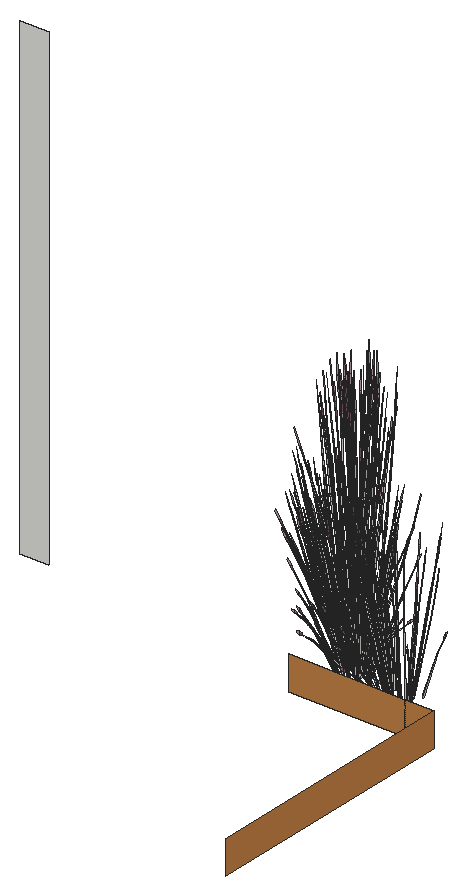
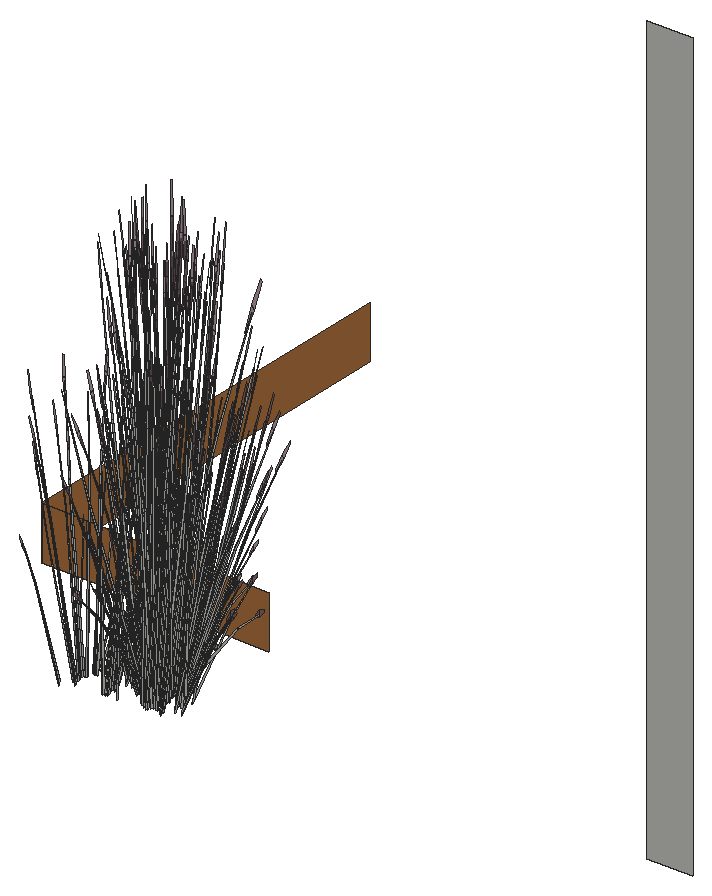
# SketchUp Ruby script. Lengths in inches.
U = 1.inch
M = Sketchup.active_model
def pt(a) = Geom::Point3d.new(a.map { |v| v * U })
def face(e, loops, mat)
  f = e.add_face(loops[0].map { |a| pt(a) })
  loops[1..].each { |l| e.add_face(l.map { |a| pt(a) }).erase! }
  f.material = f.back_material = mat if mat
  f
end
# faces: each face lists its corners as indices into pts; further lists are holes
def faces(e, pts, list, mat = nil) = list.each { |f| face(e, (f[0].is_a?(Array) ? f : [f]).map { |l| l.map { |i| pts[i] } }, mat) }
# xy, xz, yz: faces in a plane at the given z, y or x. An outline is a flat list of corners, or four numbers for a rectangle; further outlines are holes
def ring(l) = l.size == 4 ? [[l[0], l[1]], [l[2], l[1]], [l[2], l[3]], [l[0], l[3]]] : l.each_slice(2).to_a
def flat(e, list, mat, &to3) = list.each { |f| face(e, (f[0].is_a?(Array) ? f : [f]).map { |l| ring(l).map { |u, v| to3.(u, v) } }, mat) }
def xy(e, z, list, mat = nil) = flat(e, list, mat) { |x, y| [x, y, z] }
def xz(e, y, list, mat = nil) = flat(e, list, mat) { |x, z| [x, y, z] }
def yz(e, x, list, mat = nil) = flat(e, list, mat) { |y, z| [x, y, z] }
def lines(e, pts, list) = list.each { |a, b| e.add_line(pt(pts[a]), pt(pts[b])) }
# prism: a flat outline (further loops are holes) pulled along v
def prism(e, loops, v, mat = nil)
  f = face(e, loops, mat); d = Geom::Vector3d.new(v.map { |x| x * U })
  f.pushpull(f.normal.samedirection?(d) ? d.length : -d.length)
end
def box(e, o, s, mat = nil) = prism(e, [[o, [o[0] + s[0], o[1], o[2]], [o[0] + s[0], o[1] + s[1], o[2]], [o[0], o[1] + s[1], o[2]]]], [0, 0, s[2]], mat)
def at(x, y, z, deg = 0) = Geom::Transformation.translation(pt([x, y, z])) * Geom::Transformation.rotation(ORIGIN, Z_AXIS, deg.degrees)
def axes(o, x, y, z) = Geom::Transformation.new([*x, 0, *y, 0, *z, 0, *pt(o).to_a, 1])
def part(name) = M.definitions.add(name)
# library, detail: a bought-in or finely detailed component or shape, given as its bounding box
def library(name, o, s) = part(name).tap { |d| box(d.entities, o, s) }
def detail(e, o, s) = box(e.add_group.entities, o, s)
def put(e, d, t, mat = nil) = e.add_instance(d, t).tap { |i| i.material = mat if mat }
def group(e, t, mat = nil) = e.add_group.tap { |g| g.transformation = t; g.material = mat if mat }.entities
root = M.entities
M.materials.add("LightPink_Translucent").color = [144, 107, 117]
M.materials["LightPink_Translucent"].alpha = 0.75
M.materials.add("Wood_Floor_01_1K").color = [196, 130, 70]
c1 = part("blade")
p = [[2.15,0.21,22],[0,0.17,0],[0.09,0.45,0],[2.18,0.31,22],[2.29,0.31,22],[0.38,0.45,0],
  [2.48,0.24,33],[2.49,0.24,33],[2.48,0.22,33]]
faces(c1.entities,p,[[0,1,2,3],[4,5,2,3],[6,3,4,7],[8,0,3,6]])
c2 = part("seeds")
p = [[0.3,-0.1,1.38],[-0.01,-0.03,1.59],[-0.01,-0.03,0.03],[0.14,-0.07,-0.07],[0.29,-0.03,3],[0.15,0.01,3.11]]
faces(c2.entities,p,[[0,1,2,3],[1,0,4,5]],"LightPink_Translucent")
c3 = part("blade with seeds")
put(c3.entities,c1,at(0,0,0))
put(c3.entities,c2,axes([2.4,0.25,30.99],[1.5799,-0.05474,1.17369],[-0.12525,1.92788,0.29478],[-0.07173,-0.02425,1.56792]))
xz(root,99,[[360,157,384,164],[384,157,390,164]],"Wood_Floor_01_1K")
xz(root,108,[[297,156.54,303,255.54]])
yz(root,390,[[45,157,99,164]],"Wood_Floor_01_1K")
put(root,c3,axes([362.05,110.03,157.34],[0.11194,0.19382,1.61094],[-0.51725,0.16318,0.13026],[-0.1169,-0.30428,0.68866]))
put(root,c3,axes([371.95,108.74,154.43],[-0.0749,-0.08464,1.64448],[-0.49984,0.05366,-0.26007],[-0.07977,-0.20245,0.13189]))
put(root,c3,axes([362.91,108.74,158.13],[-0.0749,-0.08464,1.64448],[-0.49984,0.05366,-0.26007],[-0.07977,-0.20245,0.13189]))
put(root,c3,axes([364.07,109.75,156.13],[-0.13919,0.12219,1.34422],[-0.41687,-0.21387,-0.28909],[0.07727,-0.26598,0.57472]))
put(root,c3,axes([363.43,110.17,158.38],[-0.23372,-0.49086,-0.66783],[0.48111,-0.27356,0.08059],[-0.05465,-0.23717,0.9447]))
put(root,c3,axes([361.91,109.51,156.13],[-0.02965,0.19748,1.34422],[-0.43351,0.16532,-0.28909],[-0.10133,-0.25525,0.57472]))
put(root,c3,axes([363.03,109.08,155.1],[-0.08214,0.02175,1.65762],[-0.45422,-0.24483,-0.25323],[0.00762,-0.20421,0.28235]))
put(root,c3,axes([364.41,110.65,158.38],[0.01274,-0.55841,-0.66783],[0.53656,0.0375,0.08059],[0.05662,-0.23657,0.9447]))
put(root,c3,axes([374.19,109.78,154.43],[-0.00473,-0.12015,1.64448],[-0.39924,-0.34724,-0.26007],[0.06173,-0.21049,0.13189]))
put(root,c3,axes([365.15,109.78,158.13],[-0.00473,-0.12015,1.64448],[-0.39924,-0.34724,-0.26007],[0.06173,-0.21049,0.13189]))
put(root,c3,axes([363.48,109.75,157.95],[0.14763,-0.46424,-0.33289],[0.4307,0.1354,0.42977],[-0.03949,-0.18691,0.82232]))
put(root,c3,axes([363.8,110.37,157.34],[-0.09118,0.2075,1.61094],[-0.3825,-0.42941,0.13026],[0.17255,-0.26763,0.68866]))
put(root,c3,axes([374.09,109.35,154.43],[-0.04973,0.04611,1.6674],[-0.48725,-0.15557,-0.15755],[-0.01764,-0.20123,0.29507]))
put(root,c3,axes([365.05,109.35,158.12],[-0.04973,0.04611,1.6674],[-0.48725,-0.15557,-0.15755],[-0.01764,-0.20123,0.29507]))
put(root,c3,axes([363.26,110.07,158.1],[-0.48137,-0.15133,-0.48033],[0.165,-0.51886,-0.37205],[-0.04414,-0.2089,0.91906]))
put(root,c3,axes([363.56,108.77,156.3],[0.06282,0.35202,1.07969],[-0.34848,-0.19497,0.79328],[0.0375,-0.18025,0.23781]))
put(root,c3,axes([364.3,110.46,158.1],[-0.35055,-0.40562,-0.48033],[0.37031,-0.35523,-0.37205],[0.05334,-0.20609,0.91906]))
put(root,c3,axes([371.4375,108.46,154.43],[-0.00914,0.07236,1.6674],[-0.45057,0.26261,-0.15755],[-0.13259,-0.13424,0.29507]))
put(root,c3,axes([362.4,108.46,158.12],[-0.00914,0.07236,1.6674],[-0.45057,0.26261,-0.15755],[-0.13259,-0.13424,0.29507]))
put(root,c3,axes([371.34,109.75,154.79],[0.5455,-0.15516,0.50537],[0.09467,0.60867,0.4167],[-0.12829,-0.17939,1.04574]))
put(root,c3,axes([362.3,109.75,158.48],[0.5455,-0.15516,0.50537],[0.09467,0.60867,0.4167],[-0.12829,-0.17939,1.04574]))
put(root,c3,axes([372.57,109.86,154.45],[0.48252,0.15782,0.45122],[-0.165,0.51886,0.37205],[-0.029,-0.20404,0.9337]))
put(root,c3,axes([363.53,109.86,158.15],[0.48252,0.15782,0.45122],[-0.165,0.51886,0.37205],[-0.029,-0.20404,0.9337]))
put(root,c3,axes([363.67,110.05,158.43],[-0.47919,0.28106,-0.11431],[-0.23549,-0.49884,-0.63445],[-0.06322,-0.21021,0.96403]))
put(root,c3,axes([364.66,110.68,158.43],[-0.53819,-0.02991,-0.11431],[0.01471,-0.56632,-0.63445],[0.03738,-0.21811,0.96403]))
put(root,c3,axes([364.63,110.31,157.95],[0.33133,-0.31784,-0.33289],[0.31365,0.36292,0.42977],[0.04772,-0.1844,0.82232]))
put(root,c3,axes([361.76,109.2,156.3],[0.25544,0.21011,1.07969],[-0.37201,0.1263,0.79328],[-0.0796,-0.16148,0.23781]))
put(root,c3,axes([372.7,109.82,154.45],[0.36083,-0.20517,0.06044],[0.17661,0.37413,0.47584],[-0.03485,-0.16492,0.72558]))
put(root,c3,axes([363.66,109.82,158.14],[0.36083,-0.20517,0.06044],[0.17661,0.37413,0.47584],[-0.03485,-0.16492,0.72558]))
put(root,c3,axes([362.38,110.31,158.38],[-0.41756,-0.29179,-0.66783],[0.29675,-0.51132,0.08059],[-0.15128,-0.17422,0.9447]))
put(root,c3,axes([362.24,109.92,157.95],[-0.07563,-0.48625,-0.33289],[0.43235,-0.1284,0.42977],[-0.11613,-0.13934,0.82232]))
put(root,c3,axes([371.46,109.88,154.45],[0.22256,-0.38349,0.06044],[0.31694,0.22327,0.47584],[-0.10247,-0.12295,0.72558]))
put(root,c3,axes([362.42,109.88,158.14],[0.22256,-0.38349,0.06044],[0.31694,0.22327,0.47584],[-0.10247,-0.12295,0.72558]))
put(root,c3,axes([361.5625,109.83,155.1],[-0.04743,0.07953,1.65762],[-0.47936,0.17146,-0.25323],[-0.1158,-0.15598,0.28235]))
put(root,c3,axes([361.31,110.63,157.34],[0.1819,0.10401,1.61094],[-0.37643,0.43634,0.13026],[-0.23461,-0.19684,0.68866]))
put(root,c3,axes([365.04,110.12,155.1],[-0.07329,-0.04756,1.65762],[-0.18827,-0.53132,-0.25323],[0.127,-0.14418,0.28235]))
put(root,c3,axes([372.56,110.24,154.75],[-0.14763,0.46424,0.33289],[-0.4307,-0.1354,-0.42977],[-0.03949,-0.18691,0.82232]))
put(root,c3,axes([363.52,110.24,158.44],[-0.14763,0.46424,0.33289],[-0.4307,-0.1354,-0.42977],[-0.03949,-0.18691,0.82232]))
put(root,c3,axes([362.18,110.32,158.1],[-0.48321,0.1435,-0.48033],[-0.08453,-0.54345,-0.37205],[-0.12979,-0.15574,0.91906]))
put(root,c3,axes([373.67,110.4375,154.45],[0.3487,0.41189,0.45122],[-0.37031,0.35523,0.37205],[0.06432,-0.19325,0.9337]))
put(root,c3,axes([364.625,110.4375,158.15],[0.3487,0.41189,0.45122],[-0.37031,0.35523,0.37205],[0.06432,-0.19325,0.9337]))
put(root,c3,axes([371.5625,109.84,155.1],[-0.32682,0.57873,-0.12802],[-0.47329,-0.33342,-0.71058],[-0.16452,-0.16351,1.07972]))
put(root,c3,axes([362.52,109.84,158.8],[-0.32682,0.57873,-0.12802],[-0.47329,-0.33342,-0.71058],[-0.16452,-0.16351,1.07972]))
put(root,c3,axes([373.79,110.48,154.45],[0.40242,0.02813,0.06044],[-0.01103,0.42474,0.47584],[0.04211,-0.1627,0.72558]))
put(root,c3,axes([364.75,110.48,158.14],[0.40242,0.02813,0.06044],[-0.01103,0.42474,0.47584],[0.04211,-0.1627,0.72558]))
put(root,c3,axes([373.49,110.77,154.75],[-0.33133,0.31784,0.33289],[-0.31365,-0.36292,-0.42977],[0.04772,-0.1844,0.82232]))
put(root,c3,axes([364.45,110.77,158.44],[-0.33133,0.31784,0.33289],[-0.31365,-0.36292,-0.42977],[0.04772,-0.1844,0.82232]))
put(root,c3,axes([365.04,111.62,158.38],[0.25579,-0.47633,-0.66783],[0.44823,0.33852,0.08059],[0.15273,-0.17258,0.9447]))
put(root,c3,axes([362.27,110.23,155.93],[-0.30616,-0.60492,0],[0.51222,-0.33735,-0.48511],[0.11666,-0.07683,1.53889]))
put(root,c3,axes([365.03,111.4,158.1],[-0.1258,-0.55122,-0.48033],[0.4764,-0.09643,-0.37205],[0.13652,-0.14806,0.91906]))
put(root,c3,axes([362.95,109.51,155.7],[-0.3384,0.34633,-0.03659],[-0.31006,-0.3793,-0.1659],[-0.02183,-0.10747,0.54722]))
put(root,c3,axes([370.31,109.67,154.43],[-0.10536,-0.00426,1.64448],[-0.33544,0.42612,-0.26007],[-0.17898,-0.08707,0.13189]))
put(root,c3,axes([361.27,109.67,158.13],[-0.10536,-0.00426,1.64448],[-0.33544,0.42612,-0.26007],[-0.17898,-0.08707,0.13189]))
put(root,c3,axes([365.25,111.79,158.43],[-0.45297,-0.33287,-0.11431],[0.26096,-0.48206,-0.63445],[0.12798,-0.16757,0.96403]))
put(root,c3,axes([363.38,113.61,156.82],[0.42317,0.24343,1.42185],[-0.41456,0.52443,0.56227],[-0.18569,-0.31082,1.19198]))
put(root,c3,axes([371.53,110.32,154.75],[0.07563,0.48625,0.33289],[-0.43235,0.1284,-0.42977],[-0.11613,-0.13934,0.82232]))
put(root,c3,axes([362.49,110.32,158.44],[0.07563,0.48625,0.33289],[-0.43235,0.1284,-0.42977],[-0.11613,-0.13934,0.82232]))
put(root,c3,axes([365.41,111.18,156.13],[-0.17494,-0.01788,1.34422],[-0.17922,-0.47967,-0.28909],[0.21491,-0.13569,0.57472]))
put(root,c3,axes([370.23,110.64,154.79],[0.4044,-0.44551,0.50537],[0.34877,0.47312,0.4167],[-0.18973,-0.08218,1.04574]))
put(root,c3,axes([361.19,110.64,158.48],[0.4044,-0.44551,0.50537],[0.34877,0.47312,0.4167],[-0.18973,-0.08218,1.04574]))
put(root,c3,axes([375.41,111.65,154.43],[-0.06396,-0.00458,1.6674],[-0.2656,-0.49127,-0.15755],[0.10666,-0.16153,0.29507]))
put(root,c3,axes([366.37,111.65,158.12],[-0.06396,-0.00458,1.6674],[-0.2656,-0.49127,-0.15755],[0.10666,-0.16153,0.29507]))
put(root,c3,axes([365.61,110.3,156.3],[-0.16311,0.3073,1.07969],[-0.1402,-0.41288,0.79328],[0.13471,-0.10346,0.23781]))
put(root,c3,axes([365.38,111.46,157.95],[0.42626,-0.08628,-0.33289],[0.11256,0.4932,0.42977],[0.12215,-0.13247,0.82232]))
put(root,c3,axes([370.42,110.63,154.45],[0.02466,-0.45905,0.06044],[0.37234,0.01259,0.47584],[-0.14263,-0.04803,0.72558]))
put(root,c3,axes([361.38,110.63,158.14],[0.02466,-0.45905,0.06044],[0.37234,0.01259,0.47584],[-0.14263,-0.04803,0.72558]))
put(root,c3,axes([362.66,112.17,155.77],[0.23759,-0.54397,-0.42055],[0.49367,0.26179,0.2024],[0,-0.12539,1.35025]))
put(root,c3,axes([361.23,110.78,157.95],[-0.27863,-0.37797,-0.33289],[0.31815,-0.35779,0.42977],[-0.16164,-0.05444,0.82232]))
put(root,c3,axes([362.875,111.9,156.2],[-0.05706,-0.68884,-0.2735],[0.59432,-0.04165,-0.47002],[0.10465,-0.09176,1.50125]))
put(root,c3,axes([361.4,111.94,155.6],[0.34183,-0.37665,-0.29119],[0.34183,0.37665,0.29119],[0,-0.12132,1.30635]))
put(root,c3,axes([361.26,110.14,155.7],[-0.14126,0.49294,-0.03659],[-0.43477,-0.15163,-0.1659],[-0.06601,-0.08063,0.54722]))
put(root,c3,axes([374.07,111.75,154.75],[-0.42626,0.08628,0.33289],[-0.11256,-0.4932,-0.42977],[0.12215,-0.13247,0.82232]))
put(root,c3,axes([365.03,111.75,158.44],[-0.42626,0.08628,0.33289],[-0.11256,-0.4932,-0.42977],[0.12215,-0.13247,0.82232]))
put(root,c3,axes([362.6,112.625,156.2],[-0.55148,-0.28805,-0.2735],[0.26554,-0.60796,-0.47002],[-0.01733,-0.14927,1.50125]))
put(root,c3,axes([361.03,112.39,155.93],[-0.61233,0,0],[0,-0.67471,-0.48511],[0,-0.15367,1.53889]))
put(root,c3,axes([361.13,111.18,156.13],[0.09561,0.16807,1.34422],[-0.22031,0.45686,-0.28909],[-0.22622,-0.1092,0.57472]))
put(root,c3,axes([362.8,110.38,155.6],[0.45686,0.14937,-0.29119],[-0.11503,0.52602,0.29119],[0.0921,-0.06066,1.30635]))
put(root,c3,axes([361.53,111.03,158.38],[-0.48951,-0.01454,-0.66783],[0.03288,-0.61207,0.08059],[-0.20738,-0.06459,0.9447]))
put(root,c3,axes([374.46,111.67,154.45],[0.33617,0.25389,0.06044],[-0.19572,0.36154,0.47584],[0.10778,-0.11689,0.72558]))
put(root,c3,axes([365.42,111.67,158.14],[0.33617,0.25389,0.06044],[-0.19572,0.36154,0.47584],[0.10778,-0.11689,0.72558]))
put(root,c3,axes([374.36,111.5625,154.45],[0.12145,0.5556,0.45122],[-0.4764,0.09643,0.37205],[0.14041,-0.13067,0.9337]))
put(root,c3,axes([365.32,111.5625,158.15],[0.12145,0.5556,0.45122],[-0.4764,0.09643,0.37205],[0.14041,-0.13067,0.9337]))
put(root,c3,axes([366.61,112.24,158.13],[0.06795,-0.09195,1.64448],[-0.08698,-0.56405,-0.26007],[0.1705,-0.10694,0.13189]))
put(root,c3,axes([361.5,112.21,155.89],[-0.45549,0.50754,0.28911],[-0.45577,-0.5022,-0.34302],[-0.01591,-0.14413,1.54992]))
put(root,c3,axes([369.9,110.03,154.43],[0.0363,0.06025,1.6674],[-0.17501,0.54156,-0.15755],[-0.17724,0.00392,0.29507]))
put(root,c3,axes([360.86,110.03,158.12],[0.0363,0.06025,1.6674],[-0.17501,0.54156,-0.15755],[-0.17724,0.00392,0.29507]))
put(root,c3,axes([362.95,112.44,155.98],[0.55175,0.29259,0.22621],[-0.26554,0.60796,0.47002],[0,-0.14015,1.5091]))
put(root,c3,axes([362.74,113.27,155.99],[0.12979,-0.71533,-0.22023],[0.6154,0.12469,0.48194],[-0.10753,-0.09879,1.47054]))
put(root,c3,axes([361.37,111.15,158.1],[-0.35558,0.39989,-0.48033],[-0.31141,-0.42243,-0.37205],[-0.18066,-0.06084,0.91906]))
put(root,c3,axes([370.67,110.98,154.75],[0.27863,0.37797,0.33289],[-0.31815,0.35779,-0.42977],[-0.16164,-0.05444,0.82232]))
put(root,c3,axes([361.63,110.98,158.44],[0.27863,0.37797,0.33289],[-0.31815,0.35779,-0.42977],[-0.16164,-0.05444,0.82232]))
put(root,c3,axes([360.57,111.68,156.3],[0.31263,-0.0432,1.07969],[-0.19831,0.38061,0.79328],[-0.15449,-0.0571,0.23781]))
put(root,c3,axes([362.77,112.04,156.25],[-0.53176,0.03727,0.42055],[-0.04809,-0.6186,-0.2024],[0.0952,-0.0627,1.35025]))
put(root,c3,axes([361.55,110.74,158.43],[-0.02622,0.61393,-0.11431],[-0.49645,-0.01678,-0.63445],[-0.1912,-0.04265,0.96403]))
put(root,c3,axes([361.4,112.49,156.03],[0,0.60368,0.46672],[-0.54787,0,0],[0,-0.13749,1.48054]))
put(root,c3,axes([365.27,113.09,158.43],[-0.24639,-0.54664,-0.11431],[0.43729,-0.26863,-0.63445],[0.18428,-0.07212,0.96403]))
put(root,c3,axes([365.25,112.62,158.1],[0.13266,-0.54912,-0.48033],[0.45484,0.18822,-0.37205],[0.18313,-0.05035,0.91906]))
put(root,c3,axes([364.53,110.39,155.93],[0.30616,-0.60492,0],[0.51222,0.33735,-0.48511],[0.11666,0.07683,1.53889]))
put(root,c3,axes([360.92,111.58,157.34],[0.20312,-0.01367,1.61094],[-0.13474,0.59258,0.13026],[-0.28946,-0.03665,0.68866]))
put(root,c3,axes([362.7,112.98,155.77],[-0.29417,-0.5067,-0.42055],[0.44558,-0.35681,0.2024],[-0.0952,-0.0627,1.35025]))
put(root,c3,axes([362.76,112.26,155.92],[0.2129,0.67504,0.43009],[-0.60833,0.23474,0.16877],[0.00743,-0.12404,1.49325]))
put(root,c3,axes([365.73,112.78,155.56],[-0.3154,0.07245,1.33088],[-0.0502,-0.57666,0.07618],[0.2209,-0.08728,0.75732]))
put(root,c3,axes([366.31,112.27,155.82],[-0.3036,-0.38602,-0.06098],[0.3325,-0.3537,-0.27651],[0.09421,-0.0249,0.91203]))
put(root,c3,axes([362.65,112.79,156.25],[-0.23759,0.54397,0.42055],[-0.49367,-0.26179,-0.2024],[0,-0.12539,1.35025]))
put(root,c3,axes([363.52,112.32,155.77],[0,-0.69851,0],[0.61233,0,0],[0,0,1.68689]))
put(root,c3,axes([364.26,110.7,156.03],[-0.4583,-0.30184,0.46672],[0.27394,-0.54125,0],[0.10438,0.06875,1.48054]))
put(root,c3,axes([365.16,112.82,158.38],[0.4303,-0.26662,-0.66783],[0.23981,0.54882,0.08059],[0.20791,-0.06234,0.9447]))
put(root,c3,axes([363.23,111.875,155.92],[-0.40602,0.54785,0.43009],[-0.48237,-0.48361,0.16877],[0.09788,-0.05467,1.49325]))
put(root,c3,axes([363.67,112.86,155.86],[-0.45549,-0.5196,-0.05763],[0.45577,-0.51991,0],[-0.01591,-0.01814,1.65037]))
put(root,c3,axes([362.53,110.97,156.02],[-0.14146,0.59996,0.16584],[-0.51766,-0.16978,0.32981],[0.08942,-0.00292,1.50782]))
put(root,c3,axes([374.14,112.93,154.75],[-0.40696,-0.16841,0.33289],[0.1187,-0.49132,-0.42977],[0.16385,-0.04505,0.82232]))
put(root,c3,axes([365.1,112.93,158.44],[-0.40696,-0.16841,0.33289],[0.1187,-0.49132,-0.42977],[0.16385,-0.04505,0.82232]))
put(root,c3,axes([369.875,112.03,154.45],[0.13835,-0.55043,0.45122],[0.45484,0.18822,0.37205],[-0.17887,0.03308,0.9337]))
put(root,c3,axes([360.84,112.03,158.15],[0.13835,-0.55043,0.45122],[0.45484,0.18822,0.37205],[-0.17887,0.03308,0.9337]))
put(root,c3,axes([362.3125,111.46,155.19],[-0.482,0.24169,1.21193],[-0.15342,-0.69348,0.47091],[0.29598,0.01154,1.37843]))
put(root,c3,axes([363.61,111.64,156.16],[0.09447,-0.53876,0.13611],[0.46155,0.09352,-0.38866],[0.084,0.05532,1.1914]))
put(root,c3,axes([369.84,111.88,154.45],[-0.17985,-0.41162,0.06044],[0.32797,-0.20147,0.47584],[-0.14457,0.03975,0.72558]))
put(root,c3,axes([360.8,111.88,158.14],[-0.17985,-0.41162,0.06044],[0.32797,-0.20147,0.47584],[-0.14457,0.03975,0.72558]))
put(root,c3,axes([362.81,112.92,155.92],[0.61893,0.12719,0.43009],[-0.12596,0.71835,0.16877],[-0.09045,-0.06936,1.49325]))
put(root,c3,axes([366.08,112.4,155.1],[-0.02559,-0.09165,1.65762],[0.1775,-0.53611,-0.25323],[0.17905,-0.00771,0.28235]))
put(root,c3,axes([360.79,112.31,155.1],[0.01242,0.09514,1.65762],[-0.25036,0.49684,-0.25323],[-0.17783,-0.02504,0.28235]))
put(root,c3,axes([363.41,111.78,156.25],[-0.29417,-0.5067,0.42055],[0.44558,-0.35681,-0.2024],[0.0952,0.0627,1.35025]))
put(root,c3,axes([361.89,114.1,155.6],[-0.11503,-0.52602,-0.29119],[0.45686,-0.14937,0.29119],[-0.0921,-0.06066,1.30635]))
put(root,c3,axes([362.48,114.07,156.02],[0.52621,-0.16023,0.16584],[0.12993,0.59629,0.32981],[-0.04693,-0.08688,1.50782]))
put(root,c3,axes([363.5625,111.82,156.2],[0.49442,-0.40079,-0.2735],[0.32878,0.56631,-0.47002],[0.12199,0.05751,1.50125]))
put(root,c3,axes([365.53,112.875,157.95],[0.40696,0.16841,-0.33289],[-0.1187,0.49132,0.42977],[0.16385,-0.04505,0.82232]))
put(root,c3,axes([360.74,112.09,157.95],[-0.40696,-0.16841,-0.33289],[0.1187,-0.49132,0.42977],[-0.16385,0.04505,0.82232]))
put(root,c3,axes([363.9375,112.47,155.77],[0.54787,0,0],[0,0.62498,0],[0,0,1.67702]))
put(root,c3,axes([363.01,113.26,156.2],[-0.49442,0.40079,-0.2735],[-0.32878,-0.56631,-0.47002],[-0.12199,-0.05751,1.50125]))
put(root,c3,axes([364.09,111.01,156.02],[-0.52621,0.16023,0.16584],[-0.12993,-0.59629,0.32981],[0.04693,0.08688,1.50782]))
put(root,c3,axes([364.42,112.26,157.34],[-0.20312,0.01367,1.61094],[0.13474,-0.59258,0.13026],[0.28946,0.03665,0.68866]))
put(root,c3,axes([364.68,110.98,155.6],[0.11503,0.52602,-0.29119],[-0.45686,0.14937,0.29119],[0.0921,0.06066,1.30635]))
put(root,c3,axes([374.51,113.08,154.45],[0.17985,0.41162,0.06044],[-0.32797,0.20147,0.47584],[0.14457,-0.03975,0.72558]))
put(root,c3,axes([365.47,113.08,158.14],[0.17985,0.41162,0.06044],[-0.32797,0.20147,0.47584],[0.14457,-0.03975,0.72558]))
put(root,c3,axes([363.76,112.15,155.93],[-0.61893,-0.12719,0.46247],[0.12596,-0.71835,0.18148],[0.09045,0.06936,1.60565]))
put(root,c3,axes([374.47,112.93,154.45],[-0.13835,0.55043,0.45122],[-0.45484,-0.18822,0.37205],[0.17887,-0.03308,0.9337]))
put(root,c3,axes([365.43,112.93,158.15],[-0.13835,0.55043,0.45122],[-0.45484,-0.18822,0.37205],[0.17887,-0.03308,0.9337]))
put(root,c3,axes([363.27,113.93,155.77],[-0.15978,-0.52046,0],[0.45625,-0.18226,0],[0,0,1.45109]))
put(root,c3,axes([362.96,113.43,156.16],[-0.09447,0.53876,0.13611],[-0.46155,-0.09352,-0.38866],[-0.084,-0.05532,1.1914]))
put(root,c3,axes([370.21,112.04,154.75],[0.40696,0.16841,0.33289],[-0.1187,0.49132,-0.42977],[-0.16385,0.04505,0.82232]))
put(root,c3,axes([361.17,112.04,158.44],[0.40696,0.16841,0.33289],[-0.1187,0.49132,-0.42977],[-0.16385,0.04505,0.82232]))
put(root,c3,axes([363.86,113.85,155.75],[0.51411,-0.20483,-0.18046],[0.18065,0.59003,0.00007],[0.05675,-0.02264,1.63463]))
put(root,c3,axes([364.04,114.1,156.02],[0.14146,-0.59996,0.16584],[0.51766,0.16978,0.32981],[-0.08942,0.00292,1.50782]))
put(root,c3,axes([363.93,112.74,155.78],[0.34183,0.38994,0],[-0.34183,0.38994,0],[0,0,1.5911]))
put(root,c3,axes([361.98,112.01,156.84],[0.13919,-0.08733,1.6644],[0.048,0.60974,0.13026],[-0.3015,0.08091,0.59487]))
put(root,c3,axes([364.85,112.57,156.02],[-0.38474,-0.43973,0.16584],[0.38772,-0.42651,0.32981],[-0.04249,0.0898,1.50782]))
put(root,c3,axes([366.39,112.97,156.3],[-0.30256,0.09966,1.07969],[0.14242,-0.41189,0.79328],[0.16051,0.02818,0.23781]))
put(root,c3,axes([363.15,114.16,155.76],[-0.49367,-0.27103,0],[0.23759,-0.56315,0],[0,0,1.52945]))
put(root,c3,axes([363.5625,113.44,156.01],[-0.47817,-0.48589,-0.23681],[0.40236,-0.54561,0.51822],[-0.12876,0.05684,1.58123]))
put(root,c3,axes([362.31,114.375,156.03],[0.4583,0.30184,0.46672],[-0.27394,0.54125,0],[-0.10438,-0.06875,1.48054]))
put(root,c3,axes([363.92,112.28,156.25],[0.23759,-0.54397,0.42055],[0.49367,0.26179,-0.2024],[0,0.12539,1.35025]))
put(root,c3,axes([375.29,114.72,154.43],[-0.04428,-0.05285,1.6674],[0.09686,-0.56651,-0.15755],[0.17442,-0.03619,0.29507]))
put(root,c3,axes([366.25,114.72,158.12],[-0.04428,-0.05285,1.6674],[0.09686,-0.56651,-0.15755],[0.17442,-0.03619,0.29507]))
put(root,c3,axes([360.49,112.42,158.13],[-0.07997,0.07838,1.64448],[0.0068,0.57266,-0.26007],[-0.1833,0.07447,0.13189]))
put(root,c3,axes([363.83,112.6,155.85],[0,0.69816,-0.05299],[-0.61233,0,0],[0,0.02194,1.68606]))
put(root,c3,axes([361.02,112.34,158.1],[-0.13266,0.54912,-0.48033],[-0.45484,-0.18822,-0.37205],[-0.18313,0.05035,0.91906]))
put(root,c3,axes([361,111.87,158.43],[0.24639,0.54664,-0.11431],[-0.43729,0.26863,-0.63445],[-0.18428,0.07212,0.96403]))
put(root,c3,axes([363.875,112.1,155.77],[0.29417,0.5067,-0.42055],[-0.44558,0.35681,0.2024],[0.0952,0.0627,1.35025]))
put(root,c3,axes([365.86,114.24,157.39],[-0.09372,-0.50747,-0.03282],[0.44299,-0.11666,-0.14882],[0.09251,0.03217,0.49085]))
put(root,c3,axes([362.04,114.6875,155.93],[-0.30616,0.60492,0],[-0.51222,-0.33735,-0.48511],[-0.11666,-0.07683,1.53889]))
put(root,c3,axes([364.72,114.23,158.43],[0.02622,-0.61393,-0.11431],[0.49645,0.01678,-0.63445],[0.1912,0.04265,0.96403]))
put(root,c3,axes([365.17,112.59,156.03],[0,-0.60368,0.46672],[0.54787,0,0],[0,0.13749,1.48054]))
put(root,c3,axes([363.79,113.04,156.25],[0.53176,-0.03727,0.42055],[0.04809,0.6186,-0.2024],[-0.0952,0.0627,1.35025]))
put(root,c3,axes([364.125,112.41,156.16],[0.45625,-0.17605,0.13611],[0.15978,0.50273,-0.38866],[0,0.11064,1.1914]))
put(root,c3,axes([373.68,113.99,154.75],[-0.27863,-0.37797,0.33289],[0.31815,-0.35779,-0.42977],[0.16164,0.05444,0.82232]))
put(root,c3,axes([364.64,113.99,158.44],[-0.27863,-0.37797,0.33289],[0.31815,-0.35779,-0.42977],[0.16164,0.05444,0.82232]))
put(root,c3,axes([363.32,113.34,155.77],[-0.53176,0.03727,-0.42055],[-0.04809,-0.6186,0.2024],[-0.0952,0.0627,1.35025]))
put(root,c3,axes([365.82,113.63,156.13],[-0.11793,-0.14847,1.34422],[0.15345,-0.49116,-0.28909],[0.23861,0.06653,0.57472]))
put(root,c3,axes([363.71,114.17,155.77],[0.49367,0.27103,0],[-0.23759,0.56315,0],[0,0,1.64456]))
put(root,c3,axes([365.15,113.86,158.13],[0.10505,-0.01021,1.64448],[0.28813,-0.469,-0.26007],[0.18685,0.06191,0.13189]))
put(root,c3,axes([363.91,114.77,155.76],[-0.30235,-0.60704,-0.04834],[0.51222,-0.33735,0.48511],[-0.12622,0.0578,1.53813]))
put(root,c3,axes([363.8,113.31,156.16],[0.36178,0.36271,0.13611],[-0.30177,0.40921,-0.38866],[-0.084,0.05532,1.1914]))
put(root,c3,axes([369.99,113.4,154.45],[-0.12145,-0.5556,0.45122],[0.4764,-0.09643,0.37205],[-0.14041,0.13067,0.9337]))
put(root,c3,axes([360.95,113.4,158.15],[-0.12145,-0.5556,0.45122],[0.4764,-0.09643,0.37205],[-0.14041,0.13067,0.9337]))
put(root,c3,axes([369.89,113.29,154.45],[-0.33617,-0.25389,0.06044],[0.19572,-0.36154,0.47584],[-0.10778,0.11689,0.72558]))
put(root,c3,axes([360.85,113.29,158.14],[-0.33617,-0.25389,0.06044],[0.19572,-0.36154,0.47584],[-0.10778,0.11689,0.72558]))
put(root,c3,axes([361.01,112.625,157.34],[0.16991,-0.12769,1.61094],[0.14304,0.59005,0.13026],[-0.26674,0.13336,0.68866]))
put(root,c3,axes([364.74,113.93,158.38],[0.48951,0.01454,-0.66783],[-0.03288,0.61207,0.08059],[0.20738,0.06459,0.9447]))
put(root,c3,axes([364.1875,114.42,156.03],[0.4583,-0.30184,0.46672],[0.27394,0.54125,0],[-0.10438,0.06875,1.48054]))
put(root,c3,axes([363.54,113.95,155.85],[0.2129,0.69353,-0.05652],[-0.60833,0.24302,0],[0.00743,0.02422,1.61843]))
put(root,c3,axes([363.77,114.7,155.6],[-0.45686,-0.14937,-0.29119],[0.11503,-0.52602,0.29119],[-0.0921,0.06066,1.30635]))
put(root,c3,axes([360.48,113.63,156.13],[0.17018,0.04956,1.34422],[0.10969,0.50618,-0.28909],[-0.23117,0.09475,0.57472]))
put(root,c3,axes([370.28,113.22,154.75],[0.42626,-0.08628,0.33289],[0.11256,0.4932,-0.42977],[-0.12215,0.13247,0.82232]))
put(root,c3,axes([361.24,113.22,158.44],[0.42626,-0.08628,0.33289],[0.11256,0.4932,-0.42977],[-0.12215,0.13247,0.82232]))
put(root,c3,axes([365.54,112.69,155.93],[0.61233,0,0],[0,0.67471,-0.48511],[0,0.15367,1.53889]))
put(root,c3,axes([368.64,113,154.43],[0.06249,0.01619,1.6674],[0.19333,0.53339,-0.15755],[-0.12793,0.14,0.29507]))
put(root,c3,axes([359.6,113,158.12],[0.06249,0.01619,1.6674],[0.19333,0.53339,-0.15755],[-0.12793,0.14,0.29507]))
